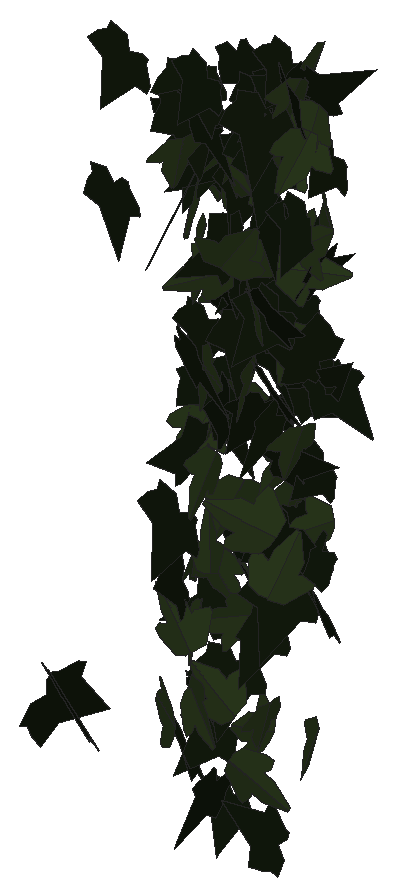
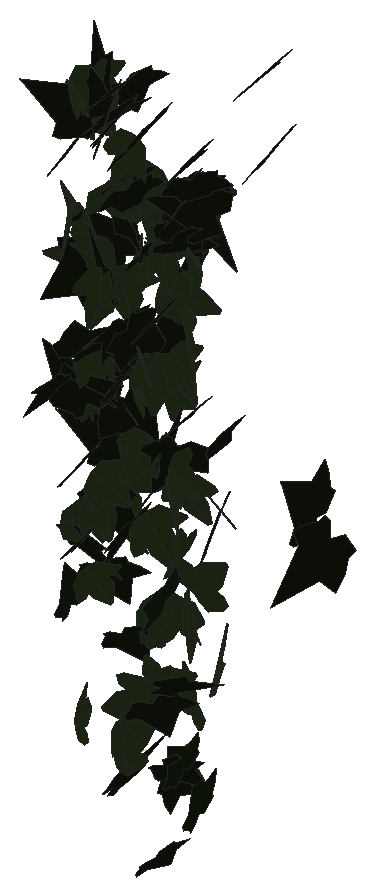
# SketchUp Ruby script. Lengths in inches.
U = 1.inch
M = Sketchup.active_model
def pt(a) = Geom::Point3d.new(a.map { |v| v * U })
def face(e, loops, mat)
  f = e.add_face(loops[0].map { |a| pt(a) })
  loops[1..].each { |l| e.add_face(l.map { |a| pt(a) }).erase! }
  f.material = f.back_material = mat if mat
  f
end
# faces: each face lists its corners as indices into pts; further lists are holes
def faces(e, pts, list, mat = nil) = list.each { |f| face(e, (f[0].is_a?(Array) ? f : [f]).map { |l| l.map { |i| pts[i] } }, mat) }
# xy, xz, yz: faces in a plane at the given z, y or x. An outline is a flat list of corners, or four numbers for a rectangle; further outlines are holes
def ring(l) = l.size == 4 ? [[l[0], l[1]], [l[2], l[1]], [l[2], l[3]], [l[0], l[3]]] : l.each_slice(2).to_a
def flat(e, list, mat, &to3) = list.each { |f| face(e, (f[0].is_a?(Array) ? f : [f]).map { |l| ring(l).map { |u, v| to3.(u, v) } }, mat) }
def xy(e, z, list, mat = nil) = flat(e, list, mat) { |x, y| [x, y, z] }
def xz(e, y, list, mat = nil) = flat(e, list, mat) { |x, z| [x, y, z] }
def yz(e, x, list, mat = nil) = flat(e, list, mat) { |y, z| [x, y, z] }
def lines(e, pts, list) = list.each { |a, b| e.add_line(pt(pts[a]), pt(pts[b])) }
# prism: a flat outline (further loops are holes) pulled along v
def prism(e, loops, v, mat = nil)
  f = face(e, loops, mat); d = Geom::Vector3d.new(v.map { |x| x * U })
  f.pushpull(f.normal.samedirection?(d) ? d.length : -d.length)
end
def box(e, o, s, mat = nil) = prism(e, [[o, [o[0] + s[0], o[1], o[2]], [o[0] + s[0], o[1] + s[1], o[2]], [o[0], o[1] + s[1], o[2]]]], [0, 0, s[2]], mat)
def at(x, y, z, deg = 0) = Geom::Transformation.translation(pt([x, y, z])) * Geom::Transformation.rotation(ORIGIN, Z_AXIS, deg.degrees)
def axes(o, x, y, z) = Geom::Transformation.new([*x, 0, *y, 0, *z, 0, *pt(o).to_a, 1])
def part(name) = M.definitions.add(name)
# library, detail: a bought-in or finely detailed component or shape, given as its bounding box
def library(name, o, s) = part(name).tap { |d| box(d.entities, o, s) }
def detail(e, o, s) = box(e.add_group.entities, o, s)
def put(e, d, t, mat = nil) = e.add_instance(d, t).tap { |i| i.material = mat if mat }
def group(e, t, mat = nil) = e.add_group.tap { |g| g.transformation = t; g.material = mat if mat }.entities
root = M.entities
M.materials.add("efeu1").color = [18, 25, 13]
M.materials.add("efeu2").color = [43, 57, 29]
c1 = part("ivyleaf_9")
p = [[1.54,2.16,1.25],[1.36,2.04,1.19],[-0.21,0.99,0.68],[-0.71,1.11,0.82],[-0.85,0.86,0.67],[-0.8,0.17,0.21],
  [-0.9,-0.01,0.1],[-0.67,-0.16,-0.02],[-0.08,-0.08,-0.05],[-0.03,-0.6,-0.4],[0.65,-0.88,-0.66],[0.83,-0.6,-0.49],
  [1.29,-0.42,-0.43],[1.8125,-0.07,-0.26],[1.21,0.44,0.15]]
faces(c1.entities,p,[[0,1,2,3,4,5,6,7,8,9,10,11,12,13,14]],"efeu1")
c2 = part("ivyleaf_10")
p = [[0,0.5,-0.03],[-0.0625,2.02,-0.43],[-0.19,2.01,-0.46],[-0.54,1.05,-0.29],[-0.52,0.625,-0.18],[-0.83,0.76,-0.28],
  [-1.16,0.64,-0.33],[-1.15,0.33,-0.24],[-0.77,-0.39,0.02],[-0.3,-0.51,0.16],[0.04,-0.48,0.23],[-0.02,2.01,-0.4375],
  [-0.06,2.01,-0.43],[0.04,-0.49,0.23],[0.67,-0.49,0.14],[1.38,0.36,-0.2],[1.375,0.51,-0.24],[0.81,0.65,-0.19],
  [0.62,0.59,-0.15],[0.6,1.09,-0.28],[0.5,1.23,-0.31]]
faces(c2.entities,p,[[0,1,2,3,4,5,6,7,8,9,10],[11,12,0,13,14,15,16,17,18,19,20]],"efeu2")
put(root,c1,axes([538.47,118.19,217.9],[0.49639,-0.72214,0.98745],[0.56169,-0.81214,-0.8763],[1.08676,0.7496,0.00188]))
put(root,c1,axes([537.28,118.77,217.32],[-0.04459,0.05768,-1.30468],[-0.4775,1.21433,0.07001],[1.21553,0.47914,-0.02036]))
put(root,c1,axes([536.76,123.47,238.17],[0.20019,-1.06234,0.2828],[0.06691,-0.27514,-1.08094],[1.0973,0.21059,0.01432]))
put(root,c1,axes([540.46,123.3125,232.28],[1.00553,-0.57363,-0.42942],[-0.36911,0.21958,-1.15762],[0.61417,1.07111,0.00734]))
put(root,c1,axes([539.05,124.65,223.58],[-0.13424,-1.02864,0.62561],[-0.04031,-0.62529,-1.03677],[1.20327,-0.13571,0.03507]))
put(root,c2,axes([540.53,124.82,226.24],[-0.01488,-0.76302,0.78628],[0.34564,-0.74947,-0.72075],[1.0397,0.23823,0.25086]))
put(root,c1,axes([535.8125,125.56,242.94],[-0.27048,-0.91346,0.63383],[0.05972,-0.66331,-0.93046],[1.11021,-0.18686,0.20446]))
put(root,c1,axes([538.12,126,219.7],[-0.13022,-0.2604,1.11383],[-0.08748,-1.11547,-0.27101],[1.14051,-0.1153,0.10639]))
put(root,c2,axes([540.4,124.7,230.59],[0.39685,-0.74713,-0.71349],[0.06201,0.78017,-0.78246],[1.03122,0.2406,0.32163]))
put(root,c2,axes([537.82,125.62,213.4],[-0.66629,0.74058,0.66765],[0.43712,-0.50477,0.99614],[0.89618,0.79681,0.01051]))
put(root,c2,axes([540.84,125.56,235.23],[-0.87847,-0.55676,0.57833],[0.55286,0.20201,1.03426],[-0.58206,1.03216,0.10954]))
put(root,c2,axes([538.74,125.57,217.51],[0.94982,0.14067,0.72978],[-0.71686,-0.13914,0.95983],[0.19614,-1.1897,-0.02597]))
put(root,c1,axes([542.16,126.41,232.88],[0.26161,-0.37446,0.95509],[0.67968,-0.67502,-0.45083],[0.76842,0.72456,0.0736]))
put(root,c1,axes([537.76,126.58,236.57],[-0.74551,0.61879,-0.64215],[0.49699,-0.40666,-0.96885],[-0.74044,-0.89597,-0.00375]))
put(root,c2,axes([541.51,126.85,222.78],[0.39933,0.52464,1.03967],[-0.66305,-0.80112,0.65893],[0.95735,-0.77368,0.0227]))
put(root,c2,axes([540.87,126.53,211.85],[-0.60297,0.10314,-1.02967],[1.01394,-0.17936,-0.61172],[-0.20687,-1.17967,0.00298]))
put(root,c1,axes([541.48,127.11,241.59],[-0.32212,-1.05615,-0.06929],[0.01831,0.06685,-1.10418],[1.05826,-0.32264,-0.00198]))
put(root,c1,axes([541.58,127.68,232.26],[-0.57026,-0.75318,0.37312],[-0.08649,-0.39592,-0.93138],[0.83607,-0.55468,0.15814]))
put(root,c2,axes([541.24,127.02,231.9],[-0.83531,0.70766,0.13036],[0.0894,-0.09612,1.09466],[0.71399,0.83993,0.01545]))
put(root,c2,axes([537.79,127.43,217.49],[0.67542,-0.57706,0.4926],[0.37226,-0.32263,-0.88836],[0.66112,0.77121,-0.00305]))
put(root,c1,axes([538.46,127.6875,209.8],[-0.23229,0.13684,-0.98546],[0.57165,-0.80989,-0.24721],[-0.81429,-0.60759,0.10757]))
put(root,c2,axes([537.5,127.49,213.44],[0.47863,-0.17826,1.05613],[1.03071,-0.2379,-0.50726],[0.29125,1.13485,0.05955]))
put(root,c1,axes([541.4375,127.83,208.12],[-0.04104,-1.04362,-0.04959],[0.00869,-0.04997,1.04437],[-1.04476,0.04058,0.01063]))
put(root,c2,axes([542.08,126.94,220.47],[0.72057,0.6946,-0.56781],[0.41127,0.39151,1.00084],[0.79733,-0.82967,-0.00309]))
put(root,c2,axes([538.37,127.97,232.81],[-0.21305,-0.21782,1.03343],[-0.66446,-0.79181,-0.30388],[0.82092,-0.69742,0.02224]))
put(root,c2,axes([542.95,127.79,240.3],[0.63984,0.6897,-0.53895],[-0.36118,-0.40007,-0.94076],[-0.79731,0.73471,-0.00635]))
put(root,c2,axes([536.84,127.61,238.19],[-0.33945,-0.94471,0.07458],[-0.01032,-0.07553,-1.00372],[0.94759,-0.33924,0.01579]))
put(root,c1,axes([542.09,128.08,241.58],[-0.14787,-0.05844,1.06242],[0.35705,-1.01315,-0.00604],[1.00232,0.35229,0.15888]))
put(root,c1,axes([539.375,127.7,234.59],[-1.03239,0.28691,0.1811],[-0.17841,0.0343,-1.07142],[-0.28859,-1.04759,0.01452]))
put(root,c2,axes([539.12,127.69,213.6875],[0.64081,0.24218,0.89079],[-0.87635,-0.18121,0.67969],[0.29013,-1.08227,0.08553]))
put(root,c2,axes([542.41,128.09,226.82],[-0.15448,-0.97061,0.22397],[-0.01033,-0.22508,-0.98252],[0.99607,-0.15287,0.02455]))
put(root,c1,axes([540.76,128.37,228.18],[0.35365,-0.53428,0.84873],[0.51421,-0.67605,-0.63984],[0.86103,0.62318,0.03352]))
put(root,c2,axes([541.96,128.36,242.18],[-0.02855,-0.9126,0.48072],[0.09528,-0.48118,-0.90782],[1.02707,0.01927,0.09758]))
put(root,c1,axes([541.16,128.14,227.14],[-0.91332,0.19062,-0.36483],[0.35659,-0.07713,-0.93299],[-0.20562,-0.98046,0.00247]))
put(root,c2,axes([538.31,127.52,220.02],[-0.08733,0.91825,-0.43017],[-0.08038,0.42414,0.92169],[1.01083,0.11305,0.03612]))
put(root,c1,axes([537.34,127.86,224.44],[-0.78015,0.55686,0.33471],[-0.28777,0.17277,-0.95818],[-0.5825,-0.83116,0.02508]))
put(root,c2,axes([538.9375,128.71,217.13],[-0.09403,-0.14003,-1.00925],[-0.59118,-0.818,0.16857],[-0.82988,0.59859,-0.00574]))
put(root,c2,axes([539.54,128.7,228.42],[0.37265,-0.63127,0.66398],[0.36024,-0.55811,-0.73279],[0.84237,0.51793,0.01964]))
put(root,c1,axes([541.71,128.28,222.27],[0.22686,0.16561,-1.03235],[-0.78573,-0.66991,-0.28013],[-0.68978,0.81757,-0.02043]))
put(root,c1,axes([542.1,128.91,236.13],[-0.2766,-0.89027,0.39213],[0.01692,-0.41202,-0.92348],[0.97266,-0.24601,0.12758]))
put(root,c1,axes([540.52,128.59,236.28],[-0.42063,-0.24656,-0.92627],[0.94768,0.04474,-0.44227],[0.14376,-1.01632,0.20525]))
put(root,c1,axes([541.09,129.23,240.81],[-0.55097,-0.62266,0.728],[-0.18742,-0.75352,-0.78634],[0.93945,-0.51551,0.27008]))
put(root,c1,axes([540.32,128.52,227.29],[0.13854,0.62848,-0.82882],[-0.25118,-0.79118,-0.64192],[-1.00937,0.28315,0.04598]))
put(root,c1,axes([541.28,128.89,219.125],[-0.7595,-0.77644,-0.16308],[0.11283,0.11776,-1.08614],[0.78532,-0.76783,-0.00167]))
put(root,c2,axes([542.78,128.53,241.16],[1.037,-0.24997,-0.04703],[-0.04496,0.01419,-1.06669],[0.25035,1.03796,0.00325]))
put(root,c1,axes([540.98,128.45,225.03],[0.36406,-0.12693,0.98829],[0.90842,-0.39001,-0.38473],[0.40937,0.97834,-0.02516]))
put(root,c2,axes([536.96,128.02,234.625],[0.63852,-0.64671,0.75688],[-0.52441,0.54582,0.90878],[-0.84622,-0.82623,0.00793]))
put(root,c2,axes([542.22,128.8125,235.07],[0.55157,-0.3833,-0.89635],[0.76541,-0.46754,0.67093],[-0.60375,-0.94291,0.03169]))
put(root,c1,axes([540.15,129.16,238.1],[-0.19351,-0.99153,0.12935],[0.02088,-0.13573,-1.00919],[0.99972,-0.18909,0.04612]))
put(root,c1,axes([539.04,129.08,230.07],[-0.33099,-0.91874,-0.13351],[0.02916,0.13138,-0.9764],[0.92794,-0.33184,-0.01694]))
put(root,c1,axes([537.72,129.38,225.46],[-0.05197,0.02956,1.02328],[-0.1993,-1.00528,0.01892],[1.00412,-0.198,0.05672]))
put(root,c1,axes([536.32,128.89,239.3],[-0.31716,-0.84929,-0.49362],[0.17758,0.46059,-0.90657],[0.96613,-0.36347,0.00459]))
put(root,c1,axes([536.52,129.58,240.25],[-0.23281,-0.75278,0.62439],[-0.01552,-0.63891,-0.77607],[0.97791,-0.18936,0.13634]))
put(root,c1,axes([540.9375,129.58,240.03],[-0.1929,-0.03737,1.02446],[-0.09573,-1.03723,-0.05586],[1.02066,-0.10435,0.18838]))
put(root,c2,axes([541.75,128.5625,233.98],[0.00179,-0.25574,-1.11141],[1.08389,0.34606,-0.07788],[0.35471,-1.05616,0.24359]))
put(root,c1,axes([535.51,129.64,209.73],[0.12584,-0.59106,0.85278],[0.29058,-0.80458,-0.60053],[0.99607,0.30939,0.06745]))
put(root,c2,axes([538.36,129.34,222.4],[-0.46205,-0.87705,0.45616],[-0.10433,-0.45745,-0.98521],[0.98306,-0.46077,0.10984]))
put(root,c1,axes([539.74,129.43,216.64],[-0.63539,-0.64803,-0.07539],[0.05411,0.05252,-0.90756],[0.65015,-0.63769,0.00186]))
put(root,c1,axes([537.35,129.49,211.19],[-0.72797,-0.48473,0.1836],[-0.15659,-0.09608,-0.87456],[0.49412,-0.74459,-0.00667]))
put(root,c1,axes([540.67,129.78,242.27],[-0.29456,-0.83063,0.51097],[0.06362,-0.549,-0.85578],[0.97313,-0.21554,0.21061]))
put(root,c1,axes([536.66,129.13,238.79],[0.65231,-0.79787,-0.07517],[-0.04143,0.06322,-1.03056],[0.80034,0.65358,0.00792]))
put(root,c2,axes([537.8125,129.42,236.71],[-0.03811,0.03539,-1.04948],[0.7999,-0.6794,-0.05196],[-0.68031,-0.8008,-0.0023]))
put(root,c1,axes([542.68,129.86,238.77],[-0.16087,-0.71802,0.7517],[0.0317,-0.76368,-0.72268],[1.03904,-0.08787,0.13843]))
put(root,c1,axes([539.25,129.6,240.46],[0.09212,-0.969,0.27289],[0.04207,-0.27008,-0.97324],[1.00581,0.10004,0.01571]))
put(root,c1,axes([539.66,129.08,221.82],[0.44838,-0.85765,-0.3751],[-0.1642,0.3374,-0.96773],[0.92158,0.47739,0.01007]))
put(root,c2,axes([539.76,128.95,239.85],[-1.03417,0.26821,-0.24851],[0.24117,-0.06,-1.06839],[-0.27483,-1.06192,-0.0024]))
put(root,c2,axes([541.75,129.82,212.1],[0.14556,-0.23843,1.00634],[0.6364,-0.78042,-0.27695],[0.81521,0.65181,0.03652]))
put(root,c1,axes([537.27,129.08,230.98],[0.8549,-0.2956,0.49709],[0.46889,-0.16507,-0.90456],[0.33856,0.97505,-0.00243]))
put(root,c2,axes([536.56,129.29,224.875],[0.9008,0.23143,-0.43295],[-0.42482,-0.08596,-0.92983],[-0.24603,0.99574,0.02035]))
put(root,c1,axes([542.03,129.68,229.43],[-0.09732,0.05044,1.04927],[-0.9996,-0.32843,-0.07693],[0.32298,-1.00129,0.07809]))
put(root,c1,axes([537.85,129.77,214.11],[-0.52774,-0.91325,-0.1621],[0.09186,0.13412,-1.0547],[0.92297,-0.53553,0.01229]))
put(root,c2,axes([540.38,129.59,237.84],[0.68947,0.52505,-0.56863],[-0.44778,-0.35053,-0.86661],[-0.63128,0.82209,-0.00634]))
put(root,c1,axes([535.25,129.04,238.25],[0.46878,-0.01387,0.92012],[0.91802,-0.06435,-0.46868],[0.06363,1.03065,-0.01688]))
put(root,c1,axes([540.08,129.52,241.39],[0.3914,-0.9047,-0.11968],[0.00451,0.13214,-0.98413],[0.91257,0.38737,0.05619]))
put(root,c1,axes([542.23,129.67,220.78],[-1.05105,-0.0233,-0.03402],[0.03407,-0.00168,-1.0513],[0.02324,-1.0516,0.00243]))
put(root,c1,axes([537.73,129.89,232.7],[0.13122,-0.95878,0.22938],[0.06211,-0.2229,-0.96724],[0.98388,0.14194,0.03046]))
put(root,c1,axes([539.23,129.8,238.4],[-0.18552,-1.00084,-0.11203],[0.02228,0.10981,-1.01789],[1.00684,-0.18684,0.00188]))
put(root,c1,axes([537.27,130.14,236.83],[-0.09256,-0.20905,-0.99796],[0.10862,-0.99838,0.19907],[-1.01382,-0.08788,0.11244]))
put(root,c2,axes([537.19,129.26,218.77],[-0.97411,-0.16567,-0.41792],[0.41724,0.03812,-0.98765],[0.16736,-1.05929,0.02982]))
put(root,c1,axes([538.14,130.11,235.91],[-0.11526,-0.87871,0.39416],[0.00785,-0.39782,-0.88456],[0.96303,-0.10192,0.05439]))
put(root,c1,axes([535.79,129.8125,240.02],[-0.46388,-0.85031,-0.28636],[0.11379,0.26401,-0.96828],[0.88999,-0.47695,-0.02546]))
put(root,c1,axes([536.46,130.1875,237.05],[-0.4815,-0.94792,0.18575],[-0.03739,-0.18911,-1.06195],[0.96522,-0.4802,0.05153]))
put(root,c2,axes([541.89,130.2,221.7],[-0.13965,0.04739,0.94196],[-0.11391,-0.94611,0.03071],[0.93625,-0.10804,0.14424]))
put(root,c1,axes([538.13,129.65,241.9],[0.43856,-0.89447,-0.20918],[-0.02605,0.2196,-0.99361],[0.91824,0.43344,0.07172]))
put(root,c2,axes([540.99,130.04,229.91],[-0.27561,-0.83124,0.55958],[0.074,-0.59566,-0.84839],[0.9993,-0.18515,0.21715]))
put(root,c1,axes([539.63,129.87,228.98],[0.44892,-0.86585,0.1528],[0.08048,-0.13038,-0.97524],[0.87553,0.45593,0.0113]))
put(root,c1,axes([541.76,130.35,224.1875],[-0.27134,-0.6118,0.70407],[-0.03285,-0.72653,-0.64398],[0.93217,-0.20369,0.18225]))
put(root,c2,axes([536.2,129.4375,218.82],[0.24674,-0.86075,-0.33384],[-0.06911,0.32737,-0.89514],[0.92064,0.25527,0.02228]))
put(root,c2,axes([538.95,130.18,211.33],[-0.09867,0.52923,0.88057],[0.17968,-0.8621,0.53826],[1.01154,0.20476,-0.00972]))
put(root,c1,axes([540.27,129.82,233.125],[-0.24265,0.39278,0.92671],[0.3757,-0.84901,0.45822],[0.93376,0.44367,0.05645]))
put(root,c1,axes([541.95,130.2,217.81],[0.06859,-0.50346,0.80513],[0.33367,-0.74297,-0.49302],[0.88902,0.31769,0.12293]))
put(root,c2,axes([536.21,129.64,233.05],[0.52595,-0.89855,-0.15739],[-0.05036,0.1528,-1.04063],[0.91084,0.52731,0.03335]))
put(root,c2,axes([540.38,130.2,224.24],[-0.19302,-0.69607,0.67241],[-0.14051,-0.65823,-0.72173],[0.95755,-0.2369,0.02964]))
put(root,c2,axes([540.62,129.93,222.95],[-0.14145,-0.89225,0.21418],[0.03215,-0.2214,-0.90107],[0.91703,-0.12986,0.06463]))
put(root,c1,axes([535.93,130.22,211.87],[0.23402,-0.66624,0.62095],[0.34033,-0.53071,-0.69768],[0.84477,0.39837,0.10905]))
put(root,c1,axes([541.59,129.71,227.46],[-0.27612,-0.13522,1.02177],[0.97491,-0.37751,0.21349],[0.33445,0.98881,0.22124]))
put(root,c2,axes([539.47,129.875,234.1],[-0.59223,-0.8143,0.204],[-0.08381,-0.19105,-1.00594],[0.83527,-0.59653,0.0437]))
put(root,c1,axes([542.06,129.59,227.99],[-0.92155,-0.20828,-0.4318],[-0.42171,-0.09281,0.94479],[-0.22801,1.01345,-0.00222]))
put(root,c2,axes([540.6,129.58,233.44],[-0.8101,-0.6012,-0.27155],[0.21346,0.16801,-1.00879],[0.6242,-0.83771,-0.00744]))
put(root,c1,axes([535.91,130.43,228.64],[-0.10458,-0.88782,0.3919],[0.10192,-0.40204,-0.88359],[0.96511,-0.05375,0.13578]))
put(root,c1,axes([536.6,129.74,226.88],[-0.31557,-0.59418,-0.764],[0.32238,0.69317,-0.67225],[0.91259,-0.45033,-0.02672]))
put(root,c1,axes([537.25,129.9,225.24],[0.51543,-0.79421,-0.18502],[-0.07965,0.1688,-0.94648],[0.81157,0.52097,0.02462]))
put(root,c2,axes([539.32,129.97,212.43],[0.00051,-0.95236,0.04986],[0.00018,-0.04986,-0.95236],[0.95366,0.00052,0.00015]))
put(root,c1,axes([542.24,128.98,233.3125],[0.23246,0.60482,0.83454],[0.32629,0.76832,-0.64771],[-0.97765,0.40024,-0.01774]))
put(root,c2,axes([541.59,130.32,242.83],[0.33589,-0.83895,0.45568],[0.19067,-0.41437,-0.90346],[0.93548,0.38569,0.02053]))
put(root,c1,axes([541.51,129.58,241.12],[0.17009,-0.12784,1.09766],[1.09873,0.13846,-0.15413],[-0.11831,1.1021,0.14669]))
put(root,c2,axes([535.93,130.61,226.24],[0.26737,-0.74185,0.71446],[0.24313,-0.67182,-0.78856],[1.00084,0.36139,0.0007]))
put(root,c2,axes([537.05,130.125,236.45],[-0.15071,-0.95944,-0.00725],[0.0029,0.00688,-0.97121],[0.95947,-0.15073,0.00179]))
put(root,c1,axes([536.98,130.65,207.43],[-0.18359,-0.88441,0.2176],[0.01733,-0.22533,-0.9012],[0.91062,-0.17401,0.06102]))
put(root,c1,axes([539.13,130.15,232.24],[0.18223,-0.92077,-0.42788],[-0.05308,0.42548,-0.93822],[1.01395,0.18776,0.02779]))
put(root,c2,axes([538.22,129.98,226.51],[-0.93509,0.18399,-0.36635],[0.35977,-0.06912,-0.95302],[-0.19654,-1.00191,-0.00152]))
put(root,c2,axes([542.33,129.75,236.38],[0.47853,-0.71819,-0.51175],[0.02263,0.59205,-0.80972],[0.88157,0.37465,0.29857]))
put(root,c2,axes([540.6,130.5625,219.64],[-0.43479,-0.6079,0.53089],[-0.02084,-0.59436,-0.69766],[0.80682,-0.34295,0.26807]))
put(root,c2,axes([536,130.47,231.64],[0.03636,-0.95414,0.32812],[0.05778,-0.32582,-0.95387],[1.00733,0.05312,0.04287]))
put(root,c2,axes([536.64,130.16,225.04],[0.46309,-0.84092,-0.16179],[-0.06397,0.14945,-0.95987],[0.85395,0.46722,0.01584]))
put(root,c2,axes([537.91,129.39,235.99],[-0.04843,0.23077,1.02772],[-0.47407,0.91394,-0.22756],[-0.94059,-0.47252,0.06178]))
put(root,c1,axes([538.3,130.83,232.39],[-0.01939,0.10838,-1.01391],[0.38087,-0.93992,-0.10776],[-0.94588,-0.38069,-0.02261]))
put(root,c2,axes([540.57,130.55,223],[-0.0421,-0.86376,0.32622],[0.08585,-0.32881,-0.85953],[0.91931,-0.00885,0.0952]))
put(root,c1,axes([536.54,130.76,215.82],[-0.66837,-0.13619,0.57994],[-0.47191,-0.4109,-0.64036],[0.36357,-0.78372,0.23496]))
put(root,c1,axes([540.71,130.24,221.86],[0.53456,-0.72192,-0.21192],[-0.0299,0.23937,-0.89086],[0.75179,0.52284,0.11525]))
put(root,c1,axes([540.25,130.99,231.06],[-0.33438,-0.80058,0.39494],[-0.04958,-0.40443,-0.8618],[0.89132,-0.32284,0.10022]))
put(root,c1,axes([536.53,130.68,219.97],[0.51182,-0.81434,0.35155],[0.18739,-0.29745,-0.96183],[0.86696,0.54504,0.00035]))
put(root,c2,axes([537.92,130.42,230.99],[0.66323,-0.85002,-0.04538],[-0.02295,0.03965,-1.07813],[0.85092,0.6636,0.00629]))
put(root,c1,axes([542.37,130.17,228.4],[0.33409,-0.7499,-0.56726],[0.04048,0.61292,-0.78641],[0.93941,0.24028,0.23562]))
put(root,c2,axes([537.35,130.32,230.78],[-0.57531,-0.8316,-0.02307],[0.02131,0.01331,-1.01115],[0.83164,-0.57561,0.00995]))
